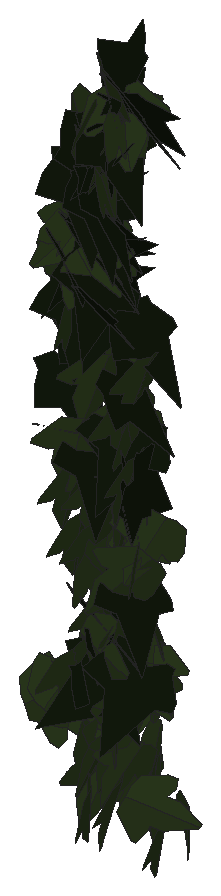
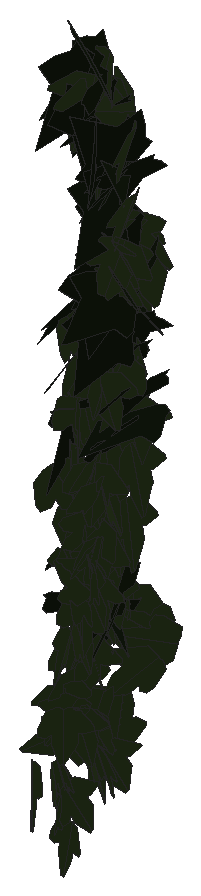
# SketchUp Ruby script. Lengths in inches.
U = 1.inch
M = Sketchup.active_model
def pt(a) = Geom::Point3d.new(a.map { |v| v * U })
def face(e, loops, mat)
  f = e.add_face(loops[0].map { |a| pt(a) })
  loops[1..].each { |l| e.add_face(l.map { |a| pt(a) }).erase! }
  f.material = f.back_material = mat if mat
  f
end
# faces: each face lists its corners as indices into pts; further lists are holes
def faces(e, pts, list, mat = nil) = list.each { |f| face(e, (f[0].is_a?(Array) ? f : [f]).map { |l| l.map { |i| pts[i] } }, mat) }
# xy, xz, yz: faces in a plane at the given z, y or x. An outline is a flat list of corners, or four numbers for a rectangle; further outlines are holes
def ring(l) = l.size == 4 ? [[l[0], l[1]], [l[2], l[1]], [l[2], l[3]], [l[0], l[3]]] : l.each_slice(2).to_a
def flat(e, list, mat, &to3) = list.each { |f| face(e, (f[0].is_a?(Array) ? f : [f]).map { |l| ring(l).map { |u, v| to3.(u, v) } }, mat) }
def xy(e, z, list, mat = nil) = flat(e, list, mat) { |x, y| [x, y, z] }
def xz(e, y, list, mat = nil) = flat(e, list, mat) { |x, z| [x, y, z] }
def yz(e, x, list, mat = nil) = flat(e, list, mat) { |y, z| [x, y, z] }
def lines(e, pts, list) = list.each { |a, b| e.add_line(pt(pts[a]), pt(pts[b])) }
# prism: a flat outline (further loops are holes) pulled along v
def prism(e, loops, v, mat = nil)
  f = face(e, loops, mat); d = Geom::Vector3d.new(v.map { |x| x * U })
  f.pushpull(f.normal.samedirection?(d) ? d.length : -d.length)
end
def box(e, o, s, mat = nil) = prism(e, [[o, [o[0] + s[0], o[1], o[2]], [o[0] + s[0], o[1] + s[1], o[2]], [o[0], o[1] + s[1], o[2]]]], [0, 0, s[2]], mat)
def at(x, y, z, deg = 0) = Geom::Transformation.translation(pt([x, y, z])) * Geom::Transformation.rotation(ORIGIN, Z_AXIS, deg.degrees)
def axes(o, x, y, z) = Geom::Transformation.new([*x, 0, *y, 0, *z, 0, *pt(o).to_a, 1])
def part(name) = M.definitions.add(name)
# library, detail: a bought-in or finely detailed component or shape, given as its bounding box
def library(name, o, s) = part(name).tap { |d| box(d.entities, o, s) }
def detail(e, o, s) = box(e.add_group.entities, o, s)
def put(e, d, t, mat = nil) = e.add_instance(d, t).tap { |i| i.material = mat if mat }
def group(e, t, mat = nil) = e.add_group.tap { |g| g.transformation = t; g.material = mat if mat }.entities
root = M.entities
M.materials.add("efeu1").color = [18, 25, 13]
M.materials.add("efeu2").color = [43, 57, 29]
c1 = part("ivyleaf_10")
p = [[0,0.5,-0.03],[-0.0625,2.02,-0.43],[-0.19,2.01,-0.46],[-0.54,1.05,-0.29],[-0.52,0.625,-0.18],[-0.83,0.76,-0.28],
  [-1.16,0.64,-0.33],[-1.15,0.33,-0.24],[-0.77,-0.39,0.02],[-0.3,-0.51,0.16],[0.04,-0.48,0.23],[-0.02,2.01,-0.4375],
  [-0.06,2.01,-0.43],[0.04,-0.49,0.23],[0.67,-0.49,0.14],[1.38,0.36,-0.2],[1.375,0.51,-0.24],[0.81,0.65,-0.19],
  [0.62,0.59,-0.15],[0.6,1.09,-0.28],[0.5,1.23,-0.31]]
faces(c1.entities,p,[[0,1,2,3,4,5,6,7,8,9,10],[11,12,0,13,14,15,16,17,18,19,20]],"efeu2")
c2 = part("ivyleaf_9")
p = [[1.54,2.16,1.25],[1.36,2.04,1.19],[-0.21,0.99,0.68],[-0.71,1.11,0.82],[-0.85,0.86,0.67],[-0.8,0.17,0.21],
  [-0.9,-0.01,0.1],[-0.67,-0.16,-0.02],[-0.08,-0.08,-0.05],[-0.03,-0.6,-0.4],[0.65,-0.88,-0.66],[0.83,-0.6,-0.49],
  [1.29,-0.42,-0.43],[1.8125,-0.07,-0.26],[1.21,0.44,0.15]]
faces(c2.entities,p,[[0,1,2,3,4,5,6,7,8,9,10,11,12,13,14]],"efeu1")
put(root,c1,axes([510.42,137.25,191.45],[-0.25135,-0.58008,-0.1738],[0.15428,0.12109,-0.64405],[0.63344,-0.25967,0.0879]))
put(root,c1,axes([510.7,137.89,186.63],[-0.54594,-0.20365,0.24936],[-0.23266,-0.1066,-0.56651],[0.24758,-0.54923,0.01749]))
put(root,c2,axes([510.4,136.87,197.82],[0.4106,0.54016,0.09943],[0.05223,0.08286,-0.68691],[-0.59014,0.38316,0.00839]))
put(root,c1,axes([510.43,136.43,199.91],[-0.67457,-0.24148,-0.16562],[0.16101,0.056,-0.69644],[0.26772,-0.64215,0.00154]))
put(root,c1,axes([510.45,137.67,190.93],[-0.5277,0.27864,-0.12476],[0.03015,-0.18516,-0.56554],[-0.32624,-0.46781,0.14953]))
put(root,c1,axes([510.55,138.41,183.5625],[-0.55956,0.24898,0.04397],[-0.06018,-0.01859,-0.59632],[-0.26603,-0.5195,0.04241]))
put(root,c2,axes([510.71,136.17,199.0625],[-0.66412,0.23401,-0.26433],[0.23298,-0.14523,-0.68187],[-0.29144,-0.64934,0.05724]))
put(root,c1,axes([510.47,136.84,192.99],[0.29017,-0.57643,0.15786],[0.07796,-0.1338,-0.66134],[0.63902,0.27807,0.00901]))
put(root,c2,axes([510.17,136.05,195.78],[0.13404,-0.72169,-0.24865],[0.04669,0.25974,-0.72869],[0.76189,0.11105,0.0884]))
put(root,c1,axes([510.56,135.86,191.91],[0.04076,-0.76332,-0.07843],[0.01673,0.0794,-0.76412],[0.76716,0.03882,0.02083]))
put(root,c1,axes([510.59,137.66,190.3],[-0.06595,-0.58038,0.21544],[-0.01305,-0.207,-0.60685],[0.66541,-0.06158,0.00945]))
put(root,c1,axes([510.625,138.21,184.53],[-0.08997,-0.51401,0.27411],[-0.04093,-0.26086,-0.54153],[0.62251,-0.09144,0.00401]))
put(root,c1,axes([510.64,137.25,193.59],[-0.6138,-0.28826,0.0147],[-0.01743,0.00059,-0.6627],[0.31121,-0.5685,-0.00814]))
put(root,c1,axes([510.625,135.5625,193.35],[-0.00279,-0.76905,0.00236],[-0.00064,-0.00236,-0.76906],[0.76906,-0.00279,-0.00063]))
put(root,c1,axes([510.53,137.28,193.22],[0.17968,0.61577,-0.09801],[-0.09566,-0.07317,-0.65983],[-0.66594,0.17665,0.06834]))
put(root,c2,axes([510.44,136.22,197.77],[-0.34512,-0.58878,-0.17028],[0.12337,0.12395,-0.69546],[0.64838,-0.33699,0.0417]))
put(root,c1,axes([510.51,135.93,201.1],[-0.17189,0.66699,0.09693],[-0.00655,0.09434,-0.71296],[-0.72732,-0.15849,-0.01649]))
put(root,c2,axes([510.44,136.55,198.64],[0.49877,0.41659,0.29136],[0.09299,0.30929,-0.62594],[-0.53415,0.44284,0.16309]))
put(root,c1,axes([510.58,135.45,197.83],[0.35076,-0.69995,-0.15253],[0.06114,0.19846,-0.77014],[0.71377,0.32697,0.14092]))
put(root,c1,axes([510.89,135.64,200.0625],[0.52856,0.26839,-0.54166],[-0.49916,-0.21209,-0.59217],[-0.34099,0.7265,0.02723]))
put(root,c1,axes([510.69,136.63,184.97],[-0.27554,-0.48772,0.34013],[0.03524,-0.36781,-0.54396],[0.63322,-0.19176,0.17828]))
put(root,c1,axes([510.65,136.85,196.16],[0.63835,0.28618,-0.13805],[-0.17238,0.02812,-0.67609],[-0.29388,0.60513,0.0967]))
put(root,c1,axes([510.37,135.4,187.26],[0.18057,0.41532,0.58566],[0.20719,0.52959,-0.46545],[-0.72675,0.25418,0.01282]))
put(root,c2,axes([510.33,136.42,196.86],[0.1885,-0.59886,-0.31066],[0.00347,0.30945,-0.64325],[0.72276,0.15471,0.08411]))
put(root,c1,axes([510.27,135.71,199.3],[-0.51337,-0.15716,-0.58973],[0.57999,0.11426,-0.53534],[0.18999,-0.77348,0.04075]))
put(root,c1,axes([510.6,136.99,185.27],[0.54132,-0.39402,0.04879],[0.02816,-0.04271,-0.66281],[0.42762,0.5016,-0.01812]))
put(root,c1,axes([510.24,134.82,187.71],[0.16511,0.1202,-0.74004],[0.58636,0.46002,0.20213],[0.51345,-0.564,0.00714]))
put(root,c1,axes([510.57,137.74,190.58],[-0.00112,-0.49378,0.38526],[0.00065,0.37045,0.51354],[-0.66668,0.00119,-0.00014]))
put(root,c1,axes([510.66,136.69,196.52],[0.05857,0.62938,0.22081],[-0.09865,0.21806,-0.64801],[-0.71055,0.02161,0.10817]))
put(root,c1,axes([510.83,137.55,189.62],[-0.66076,0.0694,0.11185],[-0.12184,-0.04432,-0.63772],[-0.06529,-0.61961,0.05814]))
put(root,c1,axes([510.65,138.67,184.53],[-0.29641,0.42633,-0.24364],[0.00268,-0.26775,-0.50978],[-0.52537,-0.2419,0.13486]))
put(root,c1,axes([510.76,136.44,198.92],[-0.7359,-0.10105,0.01011],[0.01341,-0.14841,-0.69953],[0.10882,-0.66511,0.15455]))
put(root,c1,axes([510.41,136.35,196.55],[0.65415,0.14986,0.29745],[0.22774,0.27684,-0.61529],[-0.26409,0.60994,0.20618]))
put(root,c1,axes([510.59,136.42,196.99],[-0.58936,-0.33925,-0.26119],[0.2815,0.05202,-0.6621],[0.35856,-0.59846,0.0905]))
put(root,c1,axes([510.69,137.25,190.34],[0.67549,0.0987,-0.09586],[-0.10722,0.03999,-0.65608],[-0.09887,0.63094,0.05658]))
put(root,c1,axes([510.71,136.25,185.45],[-0.18418,-0.6667,-0.28883],[-0.09255,-0.27401,0.69151],[-0.72066,0.20558,-0.01499]))
put(root,c1,axes([510.65,137.35,191.37],[-0.12372,0.60237,-0.07398],[0.00534,-0.07147,-0.63763],[-0.65506,-0.11435,0.00878]))
put(root,c1,axes([510.67,135.73,202.92],[-0.29094,0.64984,0.02255],[-0.00519,0.02148,-0.73159],[-0.7022,-0.2694,-0.00394]))
put(root,c1,axes([510.66,136.1875,199.54],[0.63834,-0.33502,0.03611],[0.04716,0.00669,-0.70601],[0.36068,0.59204,0.02841]))
put(root,c1,axes([510.75,137.65,189.15],[0.15086,-0.59244,0.09606],[0.05334,-0.08315,-0.63233],[0.64536,0.14536,0.02981]))
put(root,c1,axes([510.83,138.26,186.75],[-0.41335,-0.43154,-0.01636],[0.01117,0.01185,-0.59989],[0.46624,-0.38288,-0.00013]))
put(root,c1,axes([510.67,137.82,186.6875],[0.55451,0.30928,-0.03861],[-0.03716,-0.01482,-0.62335],[-0.33437,0.51456,0.00525]))
put(root,c1,axes([510.88,135.5,194.57],[-0.45678,-0.61046,0.15935],[-0.00649,-0.19217,-0.75481],[0.63088,-0.44397,0.10761]))
put(root,c2,axes([510.86,136.41,198.88],[0.30563,0.62624,-0.02411],[-0.01396,-0.0196,-0.71469],[-0.67666,0.28326,0.00386]))
put(root,c1,axes([510.62,134.81,187.88],[0.28714,0.40063,-0.56727],[0.29672,0.48422,0.49217],[0.62789,-0.41203,0.02683]))
put(root,c1,axes([510.9,136.01,191.72],[-0.01166,-0.75998,-0.05861],[0.00947,0.05847,-0.76002],[0.76218,-0.01235,0.00854]))
put(root,c1,axes([510.79,137.14,193.71],[-0.13253,0.63936,0.02269],[-0.03016,0.01684,-0.6766],[-0.69025,-0.12349,0.0252]))
put(root,c1,axes([510.82,137.85,187.86],[0.08067,0.59619,-0.10732],[-0.08284,-0.09381,-0.62138],[-0.64819,0.08619,0.06606]))
put(root,c1,axes([510.88,135.64,199.97],[0.65603,0.43136,-0.17251],[-0.2079,0.00564,-0.7765],[-0.41546,0.67831,0.11616]))
put(root,c2,axes([510.4,135.71,198.89],[0.12603,-0.47042,0.6314],[0.2626,-0.57772,-0.48284],[0.7423,0.28425,0.06361]))
put(root,c1,axes([510.9,136.89,185.17],[0.2733,-0.61557,-0.02002],[-0.00646,0.01835,-0.69218],[0.66511,0.25312,0.00151]))
put(root,c1,axes([510.94,136.28,189.75],[-0.02087,-0.74212,-0.0126],[-0.00061,0.01262,-0.74241],[0.74223,-0.02086,-0.00096]))
put(root,c2,axes([510.6875,135.1,194.74],[0.75935,0.27914,0.0663],[-0.08221,0.34517,-0.69873],[-0.29811,0.61585,0.36158]))
put(root,c1,axes([510.67,137.18,191.96],[-0.5173,-0.19321,-0.40778],[0.40799,0.10967,-0.53613],[0.23751,-0.6092,0.03281]))
put(root,c1,axes([510.78,136.51,186.11],[0.15992,-0.46144,0.60436],[0.24373,-0.55388,-0.4874],[0.72026,0.28989,0.03075]))
put(root,c1,axes([510.99,135.13,188.8],[-0.17056,-0.75449,-0.19553],[0.05912,0.18706,-0.77336],[0.77717,-0.17981,0.01591]))
put(root,c1,axes([510.68,136.34,199.86],[0.69482,0.06426,0.22311],[0.22431,0.07286,-0.67046],[-0.09046,0.67425,0.05118]))
put(root,c1,axes([510.76,137.3,191.46],[0.33372,-0.39662,0.41755],[0.29105,-0.29848,-0.52236],[0.53553,0.40937,0.02369]))
put(root,c1,axes([510.86,138.3,185.4],[0.456,-0.34632,0.14995],[0.12605,-0.08504,-0.56787],[0.38504,0.43799,0.00831]))
put(root,c1,axes([510.8,137.95,187.02],[0.25534,0.4611,0.32586],[0.11981,0.29462,-0.53797],[-0.59004,0.25937,0.03178]))
put(root,c1,axes([510.93,138.09,187.47],[0.40768,0.45616,-0.06458],[-0.04538,-0.04583,-0.61577],[-0.49513,0.3798,0.00326]))
put(root,c1,axes([510.96,135.73,191.11],[0.0988,-0.5842,-0.47304],[0.14918,0.48285,-0.56517],[0.73675,-0.01943,0.17787]))
put(root,c2,axes([510.97,135.87,189.17],[0.5309,-0.23892,-0.52743],[-0.45409,0.27219,-0.58038],[0.35926,0.69711,0.04585]))
put(root,c1,axes([511.06,137.88,188.83],[-0.45949,0.42749,0.05656],[-0.03563,0.04389,-0.6272],[-0.46404,-0.42666,-0.00785]))
put(root,c1,axes([511.2,135.9,193.12],[-0.1436,-0.7494,0.01594],[-0.00537,-0.0152,-0.76303],[0.74955,-0.14368,-0.00241]))
put(root,c1,axes([511.07,137.48,191.04],[0.66519,0.07933,-0.06178],[-0.06603,0.00985,-0.64559],[-0.08424,0.61869,0.0182]))
put(root,c1,axes([511.1875,136.71,186.18],[0.01315,-0.67465,0.2926],[0.0182,-0.29226,-0.67469],[0.73515,0.01931,0.01147]))
put(root,c2,axes([511.21,135.56,200.66],[0.32752,0.64045,0.36642],[0.02181,0.39232,-0.70521],[-0.73754,0.296,0.14186]))
put(root,c1,axes([511.3,135.84,196.27],[-0.27819,-0.69054,0.23758],[-0.03802,-0.24019,-0.74266],[0.72928,-0.27594,0.0519]))
put(root,c2,axes([511.62,135.86,189.57],[-0.42585,0.61854,0.11361],[-0.04783,0.10495,-0.7507],[-0.62707,-0.42807,-0.0199]))
put(root,c2,axes([511.03,136.04,194],[-0.03473,-0.77013,0.0127],[-0.00977,-0.01227,-0.77086],[0.77017,-0.03488,-0.00921]))
put(root,c2,axes([510.72,136.01,189.57],[0.46987,-0.4176,0.39503],[0.30473,-0.25448,-0.62709],[0.52805,0.51845,0.01038]))
put(root,c1,axes([511.34,135.1875,185.2],[0.3339,-0.61222,-0.24156],[-0.00857,0.2668,-0.68804],[0.65809,0.31409,0.1136]))
put(root,c2,axes([511.1,135.52,200.43],[0.77276,0.15477,-0.17109],[-0.17198,-0.01221,-0.78782],[-0.15378,0.79138,0.02131]))
put(root,c2,axes([511.125,135.52,201.6],[-0.11673,-0.78873,-0.13775],[0.07083,0.12848,-0.79572],[0.79753,-0.12685,0.05051]))
put(root,c2,axes([510.82,135.67,199.64],[0.53595,-0.52969,0.2753],[0.22748,-0.16085,-0.75232],[0.55192,0.58066,0.04274]))
put(root,c2,axes([511.125,135.81,188.51],[0.29003,-0.61027,-0.36689],[-0.10272,0.35616,-0.67361],[0.70462,0.30312,0.05282]))
put(root,c2,axes([511.26,135.47,201.97],[-0.23555,-0.17537,0.75681],[0.61003,0.44791,0.29366],[-0.48101,0.65392,0.00181]))
put(root,c2,axes([511.73,135.88,188.33],[-0.53909,-0.43006,0.3961],[-0.2975,-0.26206,-0.68941],[0.50333,-0.6155,0.01676]))
put(root,c1,axes([511.53,136.63,187.88],[-0.57782,-0.47349,0.0296],[0.09091,-0.15629,-0.72543],[0.46563,-0.55707,0.17837]))
put(root,c1,axes([511.27,135.25,199.2],[0.25373,0.68445,0.326],[0.13868,0.29607,-0.72955],[-0.74533,0.2881,-0.02476]))
put(root,c2,axes([511.98,134.96,202.1],[-0.13724,0.71433,0.35682],[-0.24864,0.30582,-0.70786],[-0.75879,-0.22941,0.16742]))
put(root,c1,axes([511.64,134.72,202.91],[0.25511,-0.36488,0.71621],[-0.28378,0.66215,0.43841],[-0.75204,-0.37363,0.07752]))
put(root,c2,axes([511.38,135.71,198.91],[-0.1237,-0.76671,0.15449],[-0.03241,-0.15125,-0.77658],[0.78144,-0.12764,-0.00776]))
put(root,c1,axes([511.66,136.54,191.125],[0.01445,-0.74954,0.00252],[0.00014,-0.00251,-0.74968],[0.74955,0.01445,0.00009]))
put(root,c2,axes([511.89,135.38,202.73],[0.10951,0.02188,-0.80908],[-0.72691,0.36171,-0.0886],[0.35594,0.73196,0.06797]))
put(root,c1,axes([511.77,136.39,185.99],[-0.19709,-0.57925,0.37893],[-0.09284,-0.36831,-0.6113],[0.68593,-0.21629,0.02614]))
put(root,c1,axes([511.8,136.25,194.92],[-0.57651,-0.47267,0.17984],[-0.03029,-0.23995,-0.72775],[0.50482,-0.55419,0.16171]))
put(root,c2,axes([511.28,135.05,198.41],[0.78751,-0.11105,0.00831],[0.00862,0.00166,-0.79529],[0.11103,0.78755,0.00285]))
put(root,c2,axes([511.37,135.59,201.15],[0.17702,-0.78367,0.04469],[0.0054,-0.04459,-0.8034],[0.78493,0.17704,-0.00455]))
put(root,c2,axes([511.5625,135.9,198.32],[-0.195,-0.71034,0.27755],[-0.00595,-0.28505,-0.73372],[0.76261,-0.18386,0.06524]))
put(root,c1,axes([511.78,136.28,189.68],[0.02415,-0.75249,-0.05337],[0.00245,0.05347,-0.75287],[0.75438,0.02392,0.00415]))
put(root,c1,axes([511.1875,135.57,189.13],[-0.14225,-0.07055,-0.7736],[0.65002,-0.44144,-0.07926],[-0.42535,-0.65102,0.13758]))
put(root,c1,axes([511.4,136.14,187.31],[0.3395,-0.32668,0.58534],[0.48433,-0.33408,-0.46736],[0.46344,0.58845,0.05962]))
put(root,c1,axes([511.77,136.2,186.98],[-0.06934,0.45006,0.60166],[0.13708,-0.5865,0.45451],[0.73875,0.15107,-0.02787]))
put(root,c1,axes([511.84,135.38,202.49],[0.20557,-0.71692,-0.33425],[0.00272,0.34599,-0.74043],[0.791,0.18513,0.08941]))
put(root,c2,axes([511.38,135.57,201.16],[0.40637,-0.68843,0.09577],[0.03596,-0.08997,-0.79928],[0.69413,0.40769,-0.01466]))
put(root,c1,axes([511.87,135.53,185.35],[0.27985,-0.70127,0.0322],[0.00791,-0.03151,-0.75503],[0.70196,0.27993,-0.00432]))
put(root,c2,axes([512.04,135.3125,203.1875],[0.16756,0.79739,-0.08508],[-0.01805,-0.08314,-0.8148],[-0.80171,0.16852,0.00057]))
put(root,c1,axes([511.97,134.95,202.08],[-0.3199,0.68504,0.29117],[-0.19975,0.22629,-0.75186],[-0.71705,-0.36866,0.07954]))
put(root,c1,axes([511.97,135.17,204.36],[-0.66575,0.4666,0.12122],[-0.10249,0.06497,-0.81297],[-0.47107,-0.67357,0.00555]))
put(root,c1,axes([511.93,136.4,193.29],[0.57528,-0.43649,-0.23143],[-0.04353,0.30907,-0.69109],[0.49213,0.53757,0.20941]))
put(root,c1,axes([511.93,136.07,194.85],[0.24852,-0.70335,-0.22325],[0.05615,0.25291,-0.73429],[0.73579,0.21826,0.13144]))
put(root,c2,axes([511.95,136.26,194.67],[-0.45634,-0.62023,0.03577],[0.02601,-0.06342,-0.76779],[0.62072,-0.45332,0.05848]))
put(root,c2,axes([512.49,135.14,204.48],[-0.23215,0.48026,0.63359],[-0.31499,0.55048,-0.53267],[-0.72998,-0.39026,0.02835]))
put(root,c1,axes([512.33,135.84,191.34],[-0.29615,-0.45272,0.59647],[-0.31122,-0.50899,-0.54084],[0.68108,-0.42943,0.01222]))
put(root,c1,axes([512.16,135.66,195.54],[-0.16201,-0.75138,-0.14465],[0.01613,0.14447,-0.76851],[0.765,-0.16218,-0.01443]))
put(root,c1,axes([512.24,135.84,191.79],[0.3336,-0.50102,-0.47557],[-0.12677,0.47475,-0.58908],[0.67905,0.33477,0.12367]))
put(root,c1,axes([512.17,136.86,183.9375],[0.26101,-0.66081,-0.1576],[-0.02406,0.15973,-0.70961],[0.67892,0.25971,0.03544]))
put(root,c2,axes([512.3,135.38,193.84],[0.3104,-0.10777,-0.72803],[-0.66692,0.29293,-0.32771],[0.31121,0.73523,0.02385]))
put(root,c2,axes([511.87,135.44,202.98],[0.17243,-0.77271,-0.18191],[0.03963,0.1943,-0.78777],[0.79285,0.15834,0.07894]))
put(root,c1,axes([512.28,135.67,194.03],[0.20281,-0.74123,0.10891],[0.02524,-0.106,-0.76847],[0.74877,0.20435,-0.00359]))
put(root,c2,axes([512.01,136.15,190.72],[0.044,-0.75772,-0.04526],[-0.00792,0.04488,-0.75897],[0.75902,0.04439,-0.00529]))
put(root,c1,axes([512.16,135.31,203.78],[0.60884,0.5261,0.15581],[0.09412,0.12915,-0.80387],[-0.54055,0.61505,0.03552]))
put(root,c1,axes([512.34,135.28,203.5],[0.04998,0.77008,0.28288],[-0.11081,0.28714,-0.76212],[-0.81288,0.00821,0.12128]))
put(root,c1,axes([512.45,137.42,184.16],[0.46352,-0.44354,-0.28824],[-0.04146,0.35161,-0.60772],[0.52735,0.4175,0.20558]))
put(root,c2,axes([512.16,135.34,196.49],[0.49466,-0.49057,-0.37121],[-0.17666,0.34299,-0.68869],[0.58928,0.51463,0.10514]))
put(root,c1,axes([512.67,136.15,192.33],[-0.47377,-0.43475,0.39921],[-0.13673,-0.41715,-0.61655],[0.57418,-0.45806,0.18259]))
put(root,c2,axes([512.11,136.0625,197.76],[0.31354,-0.67539,-0.23782],[0.00468,0.26155,-0.7366],[0.71602,0.29404,0.10895]))
put(root,c2,axes([512.56,135.77,188.77],[-0.50771,-0.58128,0.01043],[-0.00994,-0.00518,-0.77177],[0.58128,-0.50779,-0.00408]))
put(root,c2,axes([512.65,135.34,193.92],[0.15851,-0.09878,-0.78481],[-0.57733,0.5327,-0.18365],[0.54071,0.59773,0.03398]))
put(root,c1,axes([512.62,135.67,196.73],[0.08572,-0.76934,0.19742],[0.01925,-0.19649,-0.77409],[0.79403,0.08781,-0.00254]))
put(root,c2,axes([512.35,135.2,203.9],[0.76846,0.28256,-0.05523],[-0.06773,0.02441,-0.81746],[-0.27983,0.77005,0.04618]))
put(root,c1,axes([512.18,136.12,185.02],[-0.22103,-0.26492,-0.64104],[0.61256,0.24108,-0.31084],[0.3254,-0.63377,0.14972]))
put(root,c2,axes([512.18,135.15,204.22],[0.77774,-0.2613,-0.01266],[-0.01849,-0.01528,-0.82021],[0.26095,0.7777,-0.02037]))
